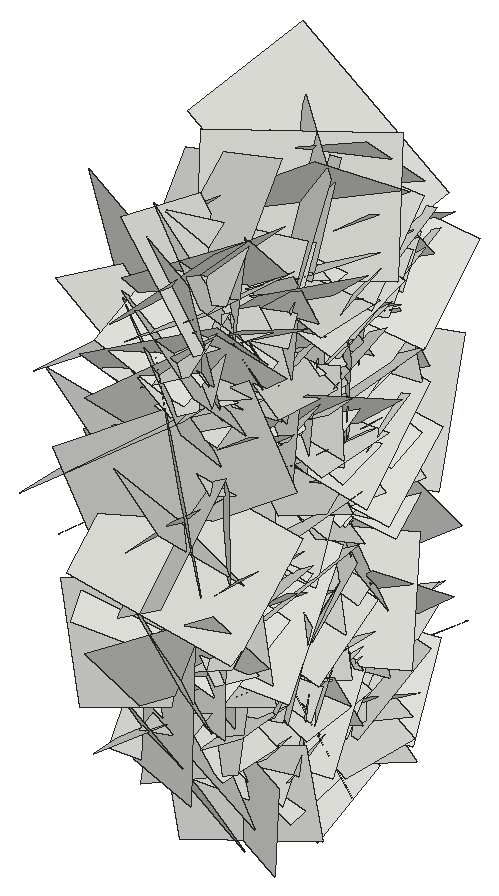
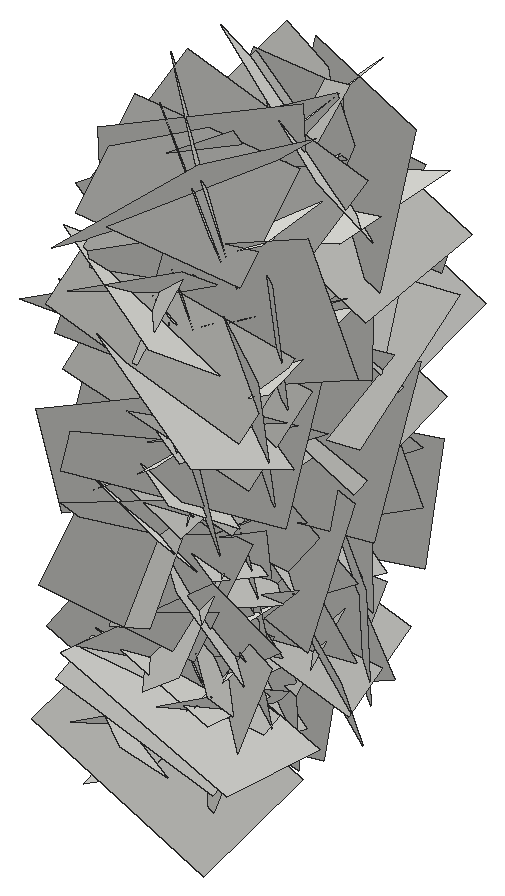
# SketchUp Ruby script. Lengths in inches.
U = 1.inch
M = Sketchup.active_model
def pt(a) = Geom::Point3d.new(a.map { |v| v * U })
def face(e, loops, mat)
  f = e.add_face(loops[0].map { |a| pt(a) })
  loops[1..].each { |l| e.add_face(l.map { |a| pt(a) }).erase! }
  f.material = f.back_material = mat if mat
  f
end
# faces: each face lists its corners as indices into pts; further lists are holes
def faces(e, pts, list, mat = nil) = list.each { |f| face(e, (f[0].is_a?(Array) ? f : [f]).map { |l| l.map { |i| pts[i] } }, mat) }
# xy, xz, yz: faces in a plane at the given z, y or x. An outline is a flat list of corners, or four numbers for a rectangle; further outlines are holes
def ring(l) = l.size == 4 ? [[l[0], l[1]], [l[2], l[1]], [l[2], l[3]], [l[0], l[3]]] : l.each_slice(2).to_a
def flat(e, list, mat, &to3) = list.each { |f| face(e, (f[0].is_a?(Array) ? f : [f]).map { |l| ring(l).map { |u, v| to3.(u, v) } }, mat) }
def xy(e, z, list, mat = nil) = flat(e, list, mat) { |x, y| [x, y, z] }
def xz(e, y, list, mat = nil) = flat(e, list, mat) { |x, z| [x, y, z] }
def yz(e, x, list, mat = nil) = flat(e, list, mat) { |y, z| [x, y, z] }
def lines(e, pts, list) = list.each { |a, b| e.add_line(pt(pts[a]), pt(pts[b])) }
# prism: a flat outline (further loops are holes) pulled along v
def prism(e, loops, v, mat = nil)
  f = face(e, loops, mat); d = Geom::Vector3d.new(v.map { |x| x * U })
  f.pushpull(f.normal.samedirection?(d) ? d.length : -d.length)
end
def box(e, o, s, mat = nil) = prism(e, [[o, [o[0] + s[0], o[1], o[2]], [o[0] + s[0], o[1] + s[1], o[2]], [o[0], o[1] + s[1], o[2]]]], [0, 0, s[2]], mat)
def at(x, y, z, deg = 0) = Geom::Transformation.translation(pt([x, y, z])) * Geom::Transformation.rotation(ORIGIN, Z_AXIS, deg.degrees)
def axes(o, x, y, z) = Geom::Transformation.new([*x, 0, *y, 0, *z, 0, *pt(o).to_a, 1])
def part(name) = M.definitions.add(name)
# library, detail: a bought-in or finely detailed component or shape, given as its bounding box
def library(name, o, s) = part(name).tap { |d| box(d.entities, o, s) }
def detail(e, o, s) = box(e.add_group.entities, o, s)
def put(e, d, t, mat = nil) = e.add_instance(d, t).tap { |i| i.material = mat if mat }
def group(e, t, mat = nil) = e.add_group.tap { |g| g.transformation = t; g.material = mat if mat }.entities
root = M.entities
c1 = part("Component\#6")
p = [[0.01,0,0],[0,3.24,4.54],[4.32,3.24,4.54],[4.33,0,0]]
faces(c1.entities,p,[[0,1,2,3]])
put(root,c1,axes([404.88,202.95,19.72],[-0.19445,-0.3512,-1.29554],[-0.25274,-1.27827,0.38028],[-1.40021,0.2795,0.11127]))
put(root,c1,axes([404.88,194.4,9.86],[-0.11876,-1.04596,0.91618],[-0.1474,0.92297,1.03671],[-1.46651,-0.00807,-0.1784]))
put(root,c1,axes([404.88,199.09,4.9],[-0.11121,1.25407,0.182],[-0.25083,0.16003,-1.23904],[-1.31962,-0.1361,0.22018]))
put(root,c1,axes([404.88,192.59,17.15],[-0.08597,-0.32374,1.28455],[-0.18245,1.27862,0.31138],[-1.3923,-0.14756,-0.12012]))
put(root,c1,axes([404.88,193.34,3.5],[-0.3285,0.68164,0.95344],[-0.04901,0.97833,-0.71446],[-1.2414,-0.219,-0.22409]))
put(root,c1,axes([404.88,197.84,15.77],[-0.08558,0.66637,-1.22765],[-0.01617,-1.23004,-0.66667],[-1.48057,-0.02508,0.07824]))
put(root,c1,axes([404.88,196.95,13.22],[-0.12152,0.35472,1.26895],[-0.01769,1.27325,-0.35743],[-1.39654,-0.047,-0.10589]))
put(root,c1,axes([404.88,198.6875,16.83],[-0.02201,1.26014,0.56955],[-0.0456,0.56875,-1.25994],[-1.46513,-0.03663,0.03065]))
put(root,c1,axes([404.88,191.67,21.5],[-0.0579,1.33618,-0.15223],[-0.05318,-0.15428,-1.33612],[-1.42453,-0.04855,0.05606]))
put(root,c1,axes([404.88,196.26,4.8],[-0.10051,-0.43998,1.12809],[-0.21352,1.12151,0.42048],[-1.26562,-0.15427,-0.16053]))
put(root,c1,axes([404.88,201.79,17.38],[-0.19939,0.73728,-1.06028],[0.09629,-1.06126,-0.75408],[-1.36551,-0.18249,0.10164]))
put(root,c1,axes([404.88,195.52,16.87],[-0.17814,-1.09516,0.21581],[-0.19304,0.24222,1.08736],[-1.16734,0.12707,-0.21275]))
put(root,c1,axes([404.88,190.86,3.39],[-0.21383,0.32739,1.20741],[0.09698,1.22359,-0.31649],[-1.32251,0.03679,-0.21843]))
put(root,c1,axes([404.88,190.45,18.05],[-0.16537,1.24759,-0.14593],[0.05265,-0.14081,-1.25691],[-1.33042,-0.16065,-0.0316]))
put(root,c1,axes([404.88,200.21,21.54],[-0.14018,1.21556,-0.55877],[0.14242,-0.54659,-1.22085],[-1.41094,-0.17594,-0.06772]))
put(root,c1,axes([404.88,192.73,15.73],[-0.12897,1.2724,-0.23633],[0.08155,-0.22984,-1.27707],[-1.36939,-0.13352,-0.05379]))
put(root,c1,axes([404.88,200.25,4.79],[-0.06637,1.27776,-0.24675],[0.01199,-0.2465,-1.2793],[-1.3794,-0.06362,0.00075]))
put(root,c1,axes([404.88,199.38,-0.0625],[-0.15183,-0.50198,1.07326],[-0.00307,1.08122,0.50532],[-1.25594,0.05804,-0.13098]))
put(root,c1,axes([404.88,192.7,21.39],[-0.08893,0.79245,0.9015],[-0.06254,0.89988,-0.79652],[-1.27076,-0.09974,-0.02389]))
put(root,c1,axes([404.88,194.09,6.34],[-0.25898,1.07168,-0.21064],[0.01285,-0.21318,-1.09862],[-1.15764,-0.24212,0.03493]))
put(root,c1,axes([404.88,200.7,5.85],[-0.20906,1.0682,-0.14016],[-0.07965,-0.15578,-1.08152],[-1.13921,-0.18514,0.10133]))
put(root,c1,axes([404.88,198.85,12.57],[-0.15345,0.48368,1.12599],[0.09378,1.13498,-0.47617],[-1.29562,0.02486,-0.16783]))
put(root,c1,axes([404.88,195.93,15.54],[-0.04965,0.25406,1.2028],[-0.02984,1.20314,-0.25523],[-1.30276,-0.03724,-0.03999]))
put(root,c1,axes([404.88,204.42,20.53],[-0.1154,-1.25003,-0.28156],[0.14973,-0.29256,1.24425],[-1.34995,0.07441,0.16208]))
put(root,c1,axes([404.88,199.56,18.73],[-0.07364,1.07871,-0.62029],[0.05176,-0.61841,-1.08091],[-1.31797,-0.08456,-0.00779]))
put(root,c1,axes([404.88,203.04,12.11],[-0.14841,-0.94408,-0.5752],[-0.05434,-0.57362,0.95398],[-1.17058,0.14632,0.02864]))
put(root,c1,axes([404.88,200.375,7.61],[-0.26418,-0.51362,-0.84712],[-0.05211,-0.86603,0.53955],[-1.04881,0.1724,0.18657]))
put(root,c1,axes([404.88,197.84,4.84],[-0.11369,-0.36766,-0.96616],[-0.19069,-0.94989,0.38144],[-1.07906,0.2066,0.03439]))
put(root,c1,axes([404.88,197.86,18.23],[-0.19608,0.2602,-1.0463],[0.01915,-1.06069,-0.26697],[-1.14269,-0.06243,0.17507]))
put(root,c1,axes([404.88,202.25,12.93],[0.19135,-1.27912,0.12446],[-0.2118,0.09622,1.27869],[-1.34571,-0.19703,-0.18355]))
put(root,c1,axes([404.88,198.375,11.05],[0.00636,-0.47599,-1.14741],[0.03555,-1.14695,0.47597],[-1.31628,-0.03327,0.00731]))
put(root,c1,axes([404.88,200.2,14.91],[-0.20407,-0.96139,-0.18597],[-0.07393,-0.17559,0.97991],[-1.03533,0.20204,-0.03331]))
put(root,c1,axes([404.88,196.53,2.03],[-0.14871,0.38131,0.94323],[-0.09041,0.94439,-0.39446],[-1.07463,-0.13222,-0.09734]))
put(root,c1,axes([404.88,192.66,5.0625],[-0.03803,0.06475,1.02957],[-0.25075,1.00223,-0.07127],[-1.06436,-0.23842,-0.02]))
put(root,c1,axes([404.88,199.09,16.39],[-0.13116,-1.14374,0.05938],[0.13174,0.04596,1.1443],[-1.20683,0.12933,0.11846]))
put(root,c1,axes([404.88,200.08,24.34],[-0.03463,0.75517,-0.67877],[-0.20748,-0.67107,-0.73718],[-1.05612,0.10708,0.16708]))
put(root,c1,axes([400.91,199.42,15.6],[-0.03605,-0.49998,-0.38134],[-0.14474,-0.36691,0.49324],[0.65063,-0.10932,0.0886]))
put(root,c1,axes([400.91,199.74,12.37],[-0.13977,-0.41949,-0.41774],[0.0557,-0.43458,0.41982],[0.62506,-0.05508,-0.13082]))
put(root,c1,axes([404.88,197.36,24.8],[0.09794,1.0389,-0.68546],[0.01654,-0.68826,-1.04104],[-1.31923,0.0685,-0.06394]))
put(root,c1,axes([404.88,194.35,10.5],[0.1187,0.07765,-1.12146],[-0.14385,-1.11784,-0.09095],[-1.18288,0.14373,-0.10148]))
put(root,c1,axes([404.88,194.25,1.05],[-0.1707,-0.55728,0.79671],[0.04122,0.80323,0.5697],[-1.02978,0.12452,-0.10926]))
put(root,c1,axes([404.88,205.24,14.9],[0.1168,-0.46047,-1.13614],[0.0362,-1.13913,0.465],[-1.29896,-0.07315,-0.0892]))
put(root,c1,axes([404.88,200.51,5.45],[0.07717,-0.59417,-0.91785],[-0.09928,-0.91989,0.58806],[-1.15472,0.03938,-0.1119]))
put(root,c1,axes([400.91,194.11,10.49],[-0.01019,-0.66626,0.06574],[-0.1187,0.06642,0.65679],[0.69967,0.00157,0.11238]))
put(root,c1,axes([404.88,202.1,18.26],[0.1919,-1.13475,-0.09678],[-0.16378,-0.12156,1.13628],[-1.19604,-0.16542,-0.17113]))
put(root,c1,axes([404.88,198.84,9.75],[0.24721,-0.9594,-0.88495],[0.06038,-0.89063,0.98057],[-1.38221,-0.2105,-0.11544]))
put(root,c1,axes([404.88,198.93,5.125],[-0.08676,0.85287,0.14934],[-0.16568,0.13299,-0.84515],[-0.90272,-0.10637,0.14076]))
put(root,c1,axes([404.88,203.91,5.3125],[-0.18463,-0.58129,-0.78091],[0.13848,-0.80009,0.56643],[-1.02258,-0.00339,0.2177]))
put(root,c1,axes([404.88,195.28,4.79],[-0.03702,0.87634,0.85063],[0.28559,0.83554,-0.84973],[-1.26267,0.16329,-0.21713]))
put(root,c1,axes([404.88,193.71,0.46],[-0.00413,-0.52236,0.7551],[-0.18121,0.74232,0.51263],[-0.95624,-0.13842,-0.10041]))
put(root,c1,axes([404.88,192.44,8.79],[0.05887,1.04295,0.25043],[-0.00297,0.2509,-1.04431],[-1.13694,0.05335,0.0157]))
put(root,c1,axes([400.91,196.1,5.28],[-0.08762,-0.56519,-0.39893],[0.0287,-0.4041,0.56691],[0.73275,-0.05175,-0.06991]))
put(root,c1,axes([400.91,199.53,17.66],[-0.07108,0.22718,0.77768],[-0.14032,0.76678,-0.23541],[0.84726,0.14605,0.02626]))
put(root,c1,axes([400.91,201.03,8.02],[-0.03451,-0.61291,-0.20918],[0.0475,-0.21108,0.61149],[0.68484,-0.01625,-0.05296]))
put(root,c1,axes([400.91,198.53,13.8],[-0.10676,-0.41647,0.70694],[-0.09382,0.7136,0.40779],[0.86465,0.02601,0.13154]))
put(root,c1,axes([404.88,196.19,13.89],[0.03711,0.95345,-0.08325],[-0.1071,-0.07916,-0.94908],[-1.00884,0.04348,0.09769]))
put(root,c1,axes([404.88,197.24,20.32],[-0.11105,0.4932,0.81979],[0.10012,0.82599,-0.48487],[-1.00916,0.02768,-0.13831]))
put(root,c1,axes([400.91,202.56,19.21],[0.06396,-0.26998,-0.58675],[-0.04641,-0.58965,0.26682],[0.68306,-0.01478,0.07307]))
put(root,c1,axes([400.91,199.64,2.06],[-0.21894,0.61345,0.59822],[0.01858,0.61825,-0.62794],[0.90807,0.13525,0.15708]))
put(root,c1,axes([404.88,196.07,8.125],[-0.08332,-0.69698,-0.457],[-0.10667,-0.44773,0.70016],[-0.87699,0.12068,-0.04174]))
put(root,c1,axes([400.91,190.79,19.57],[0.04866,0.55121,0.30162],[0.00575,0.30207,-0.55285],[0.66601,-0.04288,-0.01726]))
put(root,c1,axes([400.91,195.85,11.01],[-0.15114,0.73817,0.19544],[0.07767,0.21113,-0.74396],[0.80568,0.11812,0.10838]))
put(root,c1,axes([404.88,202.76,13.17],[0.11284,-1.03894,-0.17524],[-0.03066,-0.17895,1.04335],[-1.11641,-0.1001,-0.04636]))
put(root,c1,axes([404.88,189.31,11.46],[-0.01967,0.80876,0.77653],[0.21901,0.76581,-0.79265],[-1.16812,0.12996,-0.16169]))
put(root,c1,axes([400.91,193.57,4.75],[0.0218,0.6351,0.02763],[0.03876,0.02642,-0.63443],[0.67273,-0.0221,0.03566]))
put(root,c1,axes([404.88,199.68,18.17],[0.10811,0.81171,0.57509],[-0.11351,0.5837,-0.80488],[-1.04835,0.0205,0.14645]))
put(root,c1,axes([400.91,202.9,8.46],[-0.28421,-0.45126,-0.90988],[-0.10984,-0.92399,0.48879],[1.07096,-0.21452,-0.19133]))
put(root,c1,axes([400.91,193.91,15.9375],[0.03263,0.61645,-0.26034],[-0.02336,-0.25954,-0.61716],[0.70894,-0.03692,-0.00835]))
put(root,c1,axes([400.91,192.26,20.51],[-0.14395,0.6641,-0.62024],[-0.10915,-0.63433,-0.65665],[0.95701,0.02754,-0.16819]))
put(root,c1,axes([400.91,199.23,1.1],[-0.00098,-0.71414,-0.15761],[-0.04174,-0.15733,0.71311],[0.77408,-0.00939,0.03826]))
put(root,c1,axes([400.91,196.5625,6.92],[0.07674,-0.09799,-0.6482],[-0.03176,-0.65195,0.09521],[0.69417,-0.019,0.07601]))
put(root,c1,axes([400.91,198.91,12.75],[-0.15355,-0.10183,1.00426],[-0.21738,0.99636,0.07145],[1.04766,0.19182,0.16201]))
put(root,c1,axes([400.91,195.68,15.75],[0.06715,-0.51242,0.33521],[0.05381,0.34023,0.51051],[0.64683,0.02489,-0.07727]))
put(root,c1,axes([400.91,200.4375,8.06],[-0.17377,0.75884,-0.49804],[-0.05898,-0.51355,-0.76415],[0.96033,0.10576,-0.13705]))
put(root,c1,axes([400.91,199.6875,17.84],[0.07891,0.44569,0.39814],[0.07493,0.39183,-0.45185],[0.62903,-0.10259,0.00388]))
put(root,c1,axes([400.91,200.03,9.27],[-0.00412,-0.60297,0.30435],[0.07057,0.30253,0.60022],[0.71247,-0.03345,-0.05769]))
put(root,c1,axes([400.91,192.95,10.8],[0.02962,0.02518,0.78508],[-0.12702,0.77652,-0.02064],[0.82287,0.11896,-0.03145]))
put(root,c1,axes([404.88,199.37,10.67],[0.09558,-1.01864,0.46326],[0.13943,0.47118,1.01047],[-1.17795,-0.02688,0.1572]))
put(root,c1,axes([400.91,198.38,4.95],[-0.02223,0.32868,-0.55446],[0.17267,-0.53404,-0.32274],[0.66105,0.15055,0.06565]))
put(root,c1,axes([400.91,192.04,10.01],[-0.12172,0.5206,-0.6372],[0.01939,-0.6416,-0.52749],[0.87198,0.08694,-0.07722]))
put(root,c1,axes([400.91,202.51,19.98],[0.06792,0.48446,-0.5602],[-0.10116,-0.55221,-0.48846],[0.77852,-0.11402,-0.01459]))
put(root,c1,axes([404.88,195.86,16.68],[-0.06531,-0.43873,0.684],[-0.07025,0.68639,0.43429],[-0.8585,-0.02279,-0.08757]))
put(root,c1,axes([400.91,202.74,-0.14],[0.03158,-0.64507,0.25861],[0.01592,0.25938,0.64528],[0.73651,0.02205,-0.02503]))
put(root,c1,axes([404.88,192.22,20.81],[-0.00161,0.62306,-0.59539],[-0.0785,-0.59329,-0.62067],[-0.91013,0.05007,0.05459]))
put(root,c1,axes([400.91,197.35,3.52],[0.03443,0.41092,0.66217],[-0.08038,0.66126,-0.40665],[0.82215,0.04744,-0.06748]))
put(root,c1,axes([400.91,195.99,4.23],[-0.18601,0.0566,0.88651],[0.05201,0.90288,-0.04793],[0.94017,-0.03875,0.17804]))
put(root,c1,axes([404.88,198.67,11.97],[0.07539,0.76068,0.50866],[-0.0723,0.51318,-0.75791],[-0.96729,0.02092,0.0963]))
put(root,c1,axes([400.91,195.9375,9.16],[0.07841,0.69576,-0.29748],[-0.09095,-0.28926,-0.69787],[0.79692,-0.10147,-0.05038]))
put(root,c1,axes([404.88,195.4375,18.11],[-0.16874,-0.51977,-0.57708],[0.05885,-0.59519,0.52076],[-0.82114,0.06415,0.15591]))
put(root,c1,axes([404.88,196.17,12.88],[0.06274,0.02618,0.84664],[-0.15393,0.83645,-0.01571],[-0.88457,-0.1437,0.06278]))
put(root,c1,axes([404.88,193.46,10.77],[-0.10152,0.90556,-0.18731],[0.17799,-0.16815,-0.89879],[-0.96391,-0.12642,-0.14624]))
put(root,c1,axes([400.91,200.82,0.59],[0.02153,-0.73416,-0.35765],[-0.0933,-0.35764,0.72915],[0.8606,-0.02041,0.08799]))
put(root,c1,axes([404.88,195.73,16.63],[0.01219,-0.78698,0.32297],[-0.05977,0.32158,0.78561],[-0.89973,-0.03203,-0.04781]))
put(root,c1,axes([404.88,196.375,20.79],[0.12547,0.87042,-0.10702],[-0.18806,-0.08199,-0.86307],[-0.91037,0.1369,0.16354]))
put(root,c1,axes([404.88,200.05,13.66],[-0.07814,0.81604,-0.08962],[0.02759,-0.08761,-0.81916],[-0.86976,-0.0761,-0.01794]))
put(root,c1,axes([404.88,198.3125,4.47],[0.08144,0.93817,-0.09306],[0.01009,-0.09413,-0.94116],[-0.99929,0.07551,-0.01709]))
put(root,c1,axes([404.88,200.41,3.58],[0.05776,-0.87144,-0.04483],[-0.06577,-0.04867,0.87073],[-0.92261,-0.05109,-0.06488]))
put(root,c1,axes([404.88,195.95,14.86],[0.17446,0.9838,0.62037],[0.19333,0.59697,-0.99508],[-1.2176,0.23574,-0.06911]))
put(root,c1,axes([404.88,194.43,21.03],[0.18864,1.08922,-0.2367],[0.12278,-0.25647,-1.09312],[-1.17512,0.14806,-0.15221]))
put(root,c1,axes([400.91,200.69,6.875],[-0.16125,-0.91938,-0.30199],[-0.04119,-0.29965,0.93182],[1.02494,-0.15668,-0.01006]))
put(root,c1,axes([404.88,193.09,19.46],[-0.07295,0.25641,0.83596],[0.12348,0.83376,-0.24615],[-0.9186,0.09171,-0.09948]))
put(root,c1,axes([404.88,196.25,20.97],[-0.03433,0.46285,-0.75346],[0.09275,-0.74858,-0.46362],[-0.93272,-0.09148,-0.01837]))
put(root,c1,axes([400.91,193.9,23.36],[0.05376,0.55183,-0.55937],[-0.04326,-0.55793,-0.55411],[0.83178,-0.06469,0.00734]))
put(root,c1,axes([404.88,193.92,18.08],[0.13809,0.41624,-1.10581],[0.27382,-1.09563,-0.38198],[-1.22215,-0.19844,-0.21052]))
put(root,c1,axes([404.88,202.38,16.09],[0.07402,-0.92988,-0.45649],[0.17154,-0.44211,0.92536],[-1.08456,-0.13339,0.1152]))
put(root,c1,axes([400.91,201.99,11.3125],[-0.07595,0.62186,-0.76254],[-0.14567,-0.76339,-0.60964],[1.03278,-0.06194,-0.14206]))
put(root,c1,axes([400.91,202.11,15.27],[0.00741,-0.76642,-0.19435],[0.02033,-0.19414,0.76626],[0.83787,0.01149,-0.01688]))
put(root,c1,axes([404.88,195.27,-1.16],[0.10176,-0.07093,0.82892],[-0.16666,0.81783,0.08819],[-0.86597,-0.16573,0.08043]))
put(root,c1,axes([404.88,196.11,19.5625],[0.1708,0.27531,1.11719],[0.21419,1.10379,-0.30115],[-1.2007,0.23607,0.1052]))
put(root,c1,axes([400.91,200.46,4.14],[0.03987,0.66432,-0.22968],[0.12809,-0.2327,-0.65325],[0.73398,0.00452,0.12648]))
put(root,c1,axes([404.88,200.85,9.74],[-0.02518,0.49854,0.49521],[-0.19267,0.47427,-0.48618],[-0.7195,-0.14445,0.11286]))
put(root,c1,axes([400.91,192.1875,23.6],[0.04344,0.89705,-0.17333],[-0.1764,-0.16328,-0.88435],[0.95226,-0.07116,-0.15591]))
put(root,c1,axes([404.88,192.1875,23.6],[-0.04344,0.89705,-0.17333],[0.1764,-0.16328,-0.88435],[-0.95226,-0.07116,-0.15591]))
put(root,c1,axes([400.91,200.85,9.74],[0.02518,0.49854,0.49521],[0.19267,0.47427,-0.48618],[0.7195,-0.14445,0.11286]))
put(root,c1,axes([404.88,200.46,4.14],[-0.03987,0.66432,-0.22968],[-0.12809,-0.2327,-0.65325],[-0.73398,0.00452,0.12648]))
put(root,c1,axes([400.91,196.11,19.5625],[-0.1708,0.27531,1.11719],[-0.21419,1.10379,-0.30115],[1.2007,0.23607,0.1052]))
put(root,c1,axes([400.91,195.27,-1.16],[-0.10176,-0.07093,0.82892],[0.16666,0.81783,0.08819],[0.86597,-0.16573,0.08043]))
put(root,c1,axes([404.88,202.11,15.27],[-0.00741,-0.76642,-0.19435],[-0.02033,-0.19414,0.76626],[-0.83787,0.01149,-0.01688]))
put(root,c1,axes([404.88,201.99,11.3125],[0.07595,0.62186,-0.76254],[0.14567,-0.76339,-0.60964],[-1.03278,-0.06194,-0.14206]))
put(root,c1,axes([400.91,202.38,16.09],[-0.07402,-0.92988,-0.45649],[-0.17154,-0.44211,0.92536],[1.08456,-0.13339,0.1152]))
put(root,c1,axes([400.91,193.92,18.08],[-0.13809,0.41624,-1.10581],[-0.27382,-1.09563,-0.38198],[1.22215,-0.19844,-0.21052]))
put(root,c1,axes([404.88,193.9,23.36],[-0.05376,0.55183,-0.55937],[0.04326,-0.55793,-0.55411],[-0.83178,-0.06469,0.00734]))
put(root,c1,axes([400.91,196.25,20.97],[0.03433,0.46285,-0.75346],[-0.09275,-0.74858,-0.46362],[0.93272,-0.09148,-0.01837]))
put(root,c1,axes([400.91,193.09,19.46],[0.07295,0.25641,0.83596],[-0.12348,0.83376,-0.24615],[0.9186,0.09171,-0.09948]))
put(root,c1,axes([404.88,200.69,6.875],[0.16125,-0.91938,-0.30199],[0.04119,-0.29965,0.93182],[-1.02494,-0.15668,-0.01006]))
put(root,c1,axes([400.91,194.43,21.03],[-0.18864,1.08922,-0.2367],[-0.12278,-0.25647,-1.09312],[1.17512,0.14806,-0.15221]))
put(root,c1,axes([400.91,195.95,14.86],[-0.17446,0.9838,0.62037],[-0.19333,0.59697,-0.99508],[1.2176,0.23574,-0.06911]))
put(root,c1,axes([400.91,200.41,3.58],[-0.05776,-0.87144,-0.04483],[0.06577,-0.04867,0.87073],[0.92261,-0.05109,-0.06488]))
put(root,c1,axes([400.91,198.3125,4.47],[-0.08144,0.93817,-0.09306],[-0.01009,-0.09413,-0.94116],[0.99929,0.07551,-0.01709]))
put(root,c1,axes([400.91,200.05,13.66],[0.07814,0.81604,-0.08962],[-0.02759,-0.08761,-0.81916],[0.86976,-0.0761,-0.01794]))
put(root,c1,axes([400.91,196.375,20.79],[-0.12547,0.87042,-0.10702],[0.18806,-0.08199,-0.86307],[0.91037,0.1369,0.16354]))
put(root,c1,axes([400.91,195.73,16.63],[-0.01219,-0.78698,0.32297],[0.05977,0.32158,0.78561],[0.89973,-0.03203,-0.04781]))
put(root,c1,axes([404.88,200.82,0.59],[-0.02153,-0.73416,-0.35765],[0.0933,-0.35764,0.72915],[-0.8606,-0.02041,0.08799]))
put(root,c1,axes([400.91,193.46,10.77],[0.10152,0.90556,-0.18731],[-0.17799,-0.16815,-0.89879],[0.96391,-0.12642,-0.14624]))
put(root,c1,axes([400.91,196.17,12.88],[-0.06274,0.02618,0.84664],[0.15393,0.83645,-0.01571],[0.88457,-0.1437,0.06278]))
put(root,c1,axes([400.91,195.4375,18.11],[0.16874,-0.51977,-0.57708],[-0.05885,-0.59519,0.52076],[0.82114,0.06415,0.15591]))
put(root,c1,axes([404.88,195.9375,9.16],[-0.07841,0.69576,-0.29748],[0.09095,-0.28926,-0.69787],[-0.79692,-0.10147,-0.05038]))
put(root,c1,axes([400.91,198.67,11.97],[-0.07539,0.76068,0.50866],[0.0723,0.51318,-0.75791],[0.96729,0.02092,0.0963]))
put(root,c1,axes([404.88,195.99,4.23],[0.18601,0.0566,0.88651],[-0.05201,0.90288,-0.04793],[-0.94017,-0.03875,0.17804]))
put(root,c1,axes([404.88,197.35,3.52],[-0.03443,0.41092,0.66217],[0.08038,0.66126,-0.40665],[-0.82215,0.04744,-0.06748]))
put(root,c1,axes([400.91,192.22,20.81],[0.00161,0.62306,-0.59539],[0.0785,-0.59329,-0.62067],[0.91013,0.05007,0.05459]))
put(root,c1,axes([404.88,202.74,-0.14],[-0.03158,-0.64507,0.25861],[-0.01592,0.25938,0.64528],[-0.73651,0.02205,-0.02503]))
put(root,c1,axes([400.91,195.86,16.68],[0.06531,-0.43873,0.684],[0.07025,0.68639,0.43429],[0.8585,-0.02279,-0.08757]))
put(root,c1,axes([404.88,202.51,19.98],[-0.06792,0.48446,-0.5602],[0.10116,-0.55221,-0.48846],[-0.77852,-0.11402,-0.01459]))
put(root,c1,axes([404.88,192.04,10.01],[0.12172,0.5206,-0.6372],[-0.01939,-0.6416,-0.52749],[-0.87198,0.08694,-0.07722]))
put(root,c1,axes([404.88,198.38,4.95],[0.02223,0.32868,-0.55446],[-0.17267,-0.53404,-0.32274],[-0.66105,0.15055,0.06565]))
put(root,c1,axes([400.91,199.37,10.67],[-0.09558,-1.01864,0.46326],[-0.13943,0.47118,1.01047],[1.17795,-0.02688,0.1572]))
put(root,c1,axes([404.88,192.95,10.8],[-0.02962,0.02518,0.78508],[0.12702,0.77652,-0.02064],[-0.82287,0.11896,-0.03145]))
put(root,c1,axes([404.88,200.03,9.27],[0.00412,-0.60297,0.30435],[-0.07057,0.30253,0.60022],[-0.71247,-0.03345,-0.05769]))
put(root,c1,axes([404.88,199.6875,17.84],[-0.07891,0.44569,0.39814],[-0.07493,0.39183,-0.45185],[-0.62903,-0.10259,0.00388]))
put(root,c1,axes([404.88,200.4375,8.06],[0.17377,0.75884,-0.49804],[0.05898,-0.51355,-0.76415],[-0.96033,0.10576,-0.13705]))
put(root,c1,axes([404.88,195.68,15.75],[-0.06715,-0.51242,0.33521],[-0.05381,0.34023,0.51051],[-0.64683,0.02489,-0.07727]))
put(root,c1,axes([404.88,198.91,12.75],[0.15355,-0.10183,1.00426],[0.21738,0.99636,0.07145],[-1.04766,0.19182,0.16201]))
put(root,c1,axes([404.88,196.5625,6.92],[-0.07674,-0.09799,-0.6482],[0.03176,-0.65195,0.09521],[-0.69417,-0.019,0.07601]))
put(root,c1,axes([404.88,199.23,1.1],[0.00098,-0.71414,-0.15761],[0.04174,-0.15733,0.71311],[-0.77408,-0.00939,0.03826]))
put(root,c1,axes([404.88,192.26,20.51],[0.14395,0.6641,-0.62024],[0.10915,-0.63433,-0.65665],[-0.95701,0.02754,-0.16819]))
put(root,c1,axes([404.88,193.91,15.9375],[-0.03263,0.61645,-0.26034],[0.02336,-0.25954,-0.61716],[-0.70894,-0.03692,-0.00835]))
put(root,c1,axes([404.88,202.9,8.46],[0.28421,-0.45126,-0.90988],[0.10984,-0.92399,0.48879],[-1.07096,-0.21452,-0.19133]))
put(root,c1,axes([400.91,199.68,18.17],[-0.10811,0.81171,0.57509],[0.11351,0.5837,-0.80488],[1.04835,0.0205,0.14645]))
put(root,c1,axes([404.88,193.57,4.75],[-0.0218,0.6351,0.02763],[-0.03876,0.02642,-0.63443],[-0.67273,-0.0221,0.03566]))
put(root,c1,axes([400.91,189.31,11.46],[0.01967,0.80876,0.77653],[-0.21901,0.76581,-0.79265],[1.16812,0.12996,-0.16169]))
put(root,c1,axes([400.91,202.76,13.17],[-0.11284,-1.03894,-0.17524],[0.03066,-0.17895,1.04335],[1.11641,-0.1001,-0.04636]))
put(root,c1,axes([404.88,195.85,11.01],[0.15114,0.73817,0.19544],[-0.07767,0.21113,-0.74396],[-0.80568,0.11812,0.10838]))
put(root,c1,axes([404.88,190.79,19.57],[-0.04866,0.55121,0.30162],[-0.00575,0.30207,-0.55285],[-0.66601,-0.04288,-0.01726]))
put(root,c1,axes([400.91,196.07,8.125],[0.08332,-0.69698,-0.457],[0.10667,-0.44773,0.70016],[0.87699,0.12068,-0.04174]))
put(root,c1,axes([404.88,199.64,2.06],[0.21894,0.61345,0.59822],[-0.01858,0.61825,-0.62794],[-0.90807,0.13525,0.15708]))
put(root,c1,axes([404.88,202.56,19.21],[-0.06396,-0.26998,-0.58675],[0.04641,-0.58965,0.26682],[-0.68306,-0.01478,0.07307]))
put(root,c1,axes([400.91,197.24,20.32],[0.11105,0.4932,0.81979],[-0.10012,0.82599,-0.48487],[1.00916,0.02768,-0.13831]))
